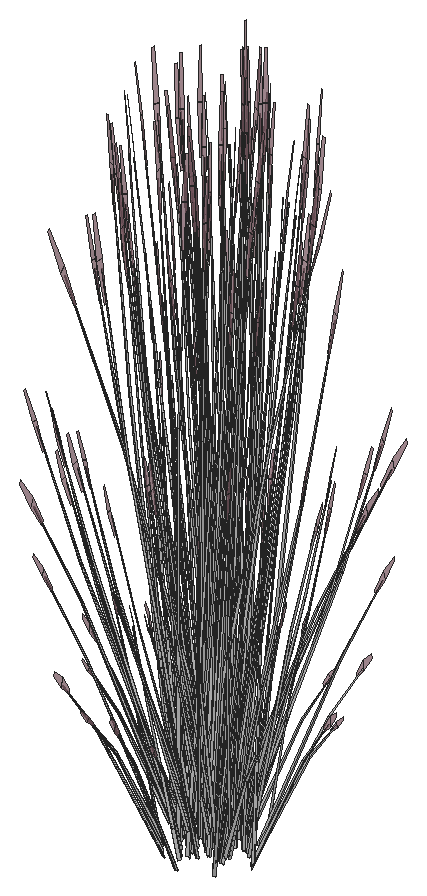
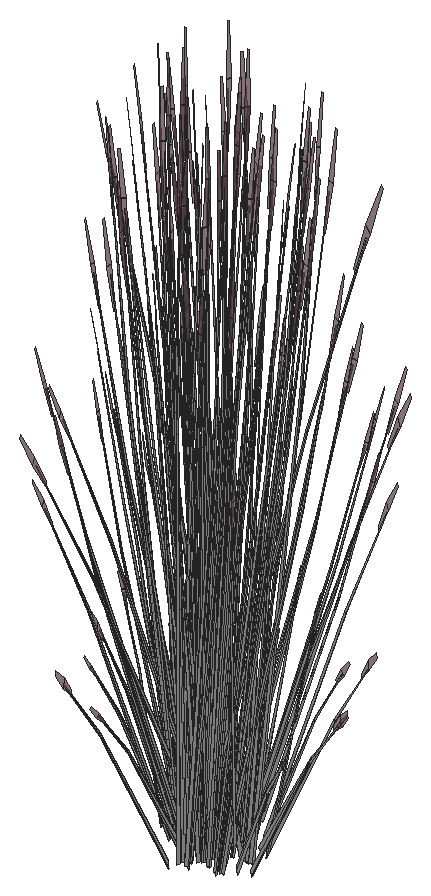
# SketchUp Ruby script. Lengths in inches.
U = 1.inch
M = Sketchup.active_model
def pt(a) = Geom::Point3d.new(a.map { |v| v * U })
def face(e, loops, mat)
  f = e.add_face(loops[0].map { |a| pt(a) })
  loops[1..].each { |l| e.add_face(l.map { |a| pt(a) }).erase! }
  f.material = f.back_material = mat if mat
  f
end
# faces: each face lists its corners as indices into pts; further lists are holes
def faces(e, pts, list, mat = nil) = list.each { |f| face(e, (f[0].is_a?(Array) ? f : [f]).map { |l| l.map { |i| pts[i] } }, mat) }
# xy, xz, yz: faces in a plane at the given z, y or x. An outline is a flat list of corners, or four numbers for a rectangle; further outlines are holes
def ring(l) = l.size == 4 ? [[l[0], l[1]], [l[2], l[1]], [l[2], l[3]], [l[0], l[3]]] : l.each_slice(2).to_a
def flat(e, list, mat, &to3) = list.each { |f| face(e, (f[0].is_a?(Array) ? f : [f]).map { |l| ring(l).map { |u, v| to3.(u, v) } }, mat) }
def xy(e, z, list, mat = nil) = flat(e, list, mat) { |x, y| [x, y, z] }
def xz(e, y, list, mat = nil) = flat(e, list, mat) { |x, z| [x, y, z] }
def yz(e, x, list, mat = nil) = flat(e, list, mat) { |y, z| [x, y, z] }
def lines(e, pts, list) = list.each { |a, b| e.add_line(pt(pts[a]), pt(pts[b])) }
# prism: a flat outline (further loops are holes) pulled along v
def prism(e, loops, v, mat = nil)
  f = face(e, loops, mat); d = Geom::Vector3d.new(v.map { |x| x * U })
  f.pushpull(f.normal.samedirection?(d) ? d.length : -d.length)
end
def box(e, o, s, mat = nil) = prism(e, [[o, [o[0] + s[0], o[1], o[2]], [o[0] + s[0], o[1] + s[1], o[2]], [o[0], o[1] + s[1], o[2]]]], [0, 0, s[2]], mat)
def at(x, y, z, deg = 0) = Geom::Transformation.translation(pt([x, y, z])) * Geom::Transformation.rotation(ORIGIN, Z_AXIS, deg.degrees)
def axes(o, x, y, z) = Geom::Transformation.new([*x, 0, *y, 0, *z, 0, *pt(o).to_a, 1])
def part(name) = M.definitions.add(name)
# library, detail: a bought-in or finely detailed component or shape, given as its bounding box
def library(name, o, s) = part(name).tap { |d| box(d.entities, o, s) }
def detail(e, o, s) = box(e.add_group.entities, o, s)
def put(e, d, t, mat = nil) = e.add_instance(d, t).tap { |i| i.material = mat if mat }
def group(e, t, mat = nil) = e.add_group.tap { |g| g.transformation = t; g.material = mat if mat }.entities
root = M.entities
M.materials.add("LightPink_Translucent").color = [144, 107, 117]
M.materials["LightPink_Translucent"].alpha = 0.75
M.materials.add("[_0053_Ivory_]").color = [200, 200, 200]
c1 = part("blade")
p = [[2.15,0.21,22],[0,0.17,0],[0.09,0.45,0],[2.18,0.31,22],[2.29,0.31,22],[0.38,0.45,0],
  [2.48,0.24,33],[2.49,0.24,33],[2.48,0.22,33]]
faces(c1.entities,p,[[0,1,2,3],[4,5,2,3],[6,3,4,7],[8,0,3,6]])
c2 = part("seeds")
p = [[0.3,-0.1,1.38],[-0.01,-0.03,1.59],[-0.01,-0.03,0.03],[0.14,-0.07,-0.07],[0.29,-0.03,3],[0.15,0.01,3.11]]
faces(c2.entities,p,[[0,1,2,3],[1,0,4,5]],"LightPink_Translucent")
c3 = part("blade with seeds")
put(c3.entities,c1,at(0,0,0))
put(c3.entities,c2,axes([2.4,0.25,30.99],[1.5799,-0.05474,1.17369],[-0.12525,1.92788,0.29478],[-0.07173,-0.02425,1.56792]))
put(root,c3,axes([642.49,106.9,130.53],[0.13883,0.2019,1.71376],[-0.64153,0.16998,0.13857],[-0.14499,-0.31697,0.73262]),"[_0053_Ivory_]")
put(root,c3,axes([644.98,106.61,129.24],[-0.17264,0.12729,1.43002],[-0.51703,-0.22279,-0.30754],[0.09584,-0.27707,0.61141]),"[_0053_Ivory_]")
put(root,c3,axes([644.2,107.05,131.63],[-0.28988,-0.51132,-0.71045],[0.59671,-0.28496,0.08574],[-0.06778,-0.24706,1.00501]),"[_0053_Ivory_]")
put(root,c3,axes([642.3125,106.37,129.24],[-0.03678,0.20572,1.43002],[-0.53767,0.17221,-0.30754],[-0.12568,-0.26589,0.61141]),"[_0053_Ivory_]")
put(root,c3,axes([643.7,105.92,128.15],[-0.10187,0.02266,1.76342],[-0.56336,-0.25503,-0.26939],[0.00945,-0.21273,0.30037]),"[_0053_Ivory_]")
put(root,c3,axes([645.4,107.55,131.63],[0.0158,-0.58168,-0.71045],[0.66548,0.03907,0.08574],[0.07023,-0.24643,1.00501]),"[_0053_Ivory_]")
put(root,c3,axes([644.25,106.62,131.18],[0.1831,-0.48359,-0.35414],[0.53419,0.14105,0.4572],[-0.04898,-0.1947,0.87481]),"[_0053_Ivory_]")
put(root,c3,axes([644.65,107.26,130.53],[-0.11309,0.21615,1.71376],[-0.47441,-0.44731,0.13857],[0.21402,-0.27879,0.73262]),"[_0053_Ivory_]")
put(root,c3,axes([643.98,106.95,131.33],[-0.59704,-0.15764,-0.51099],[0.20464,-0.54049,-0.3958],[-0.05475,-0.21761,0.97773]),"[_0053_Ivory_]")
put(root,c3,axes([644.35,105.59,129.42],[0.07791,0.3667,1.1486],[-0.43222,-0.2031,0.84392],[0.04651,-0.18776,0.25299]),"[_0053_Ivory_]")
put(root,c3,axes([645.27,107.36,131.33],[-0.43478,-0.42253,-0.51099],[0.45929,-0.37004,-0.3958],[0.06615,-0.21468,0.97773]),"[_0053_Ivory_]")
put(root,c3,axes([645.68,107.2,131.18],[0.41095,-0.33109,-0.35414],[0.38901,0.37805,0.4572],[0.05919,-0.19208,0.87481]),"[_0053_Ivory_]")
put(root,c3,axes([642.125,106.03,129.42],[0.31682,0.21887,1.1486],[-0.4614,0.13157,0.84392],[-0.09872,-0.16821,0.25299]),"[_0053_Ivory_]")
put(root,c3,axes([642.89,107.2,131.63],[-0.51789,-0.30395,-0.71045],[0.36805,-0.53263,0.08574],[-0.18764,-0.18149,1.00501]),"[_0053_Ivory_]")
put(root,c3,axes([642.71,106.79,131.18],[-0.0938,-0.50652,-0.35414],[0.53623,-0.13375,0.4572],[-0.14403,-0.14515,0.87481]),"[_0053_Ivory_]")
put(root,c3,axes([641.875,106.69,128.15],[-0.05883,0.08284,1.76342],[-0.59454,0.17861,-0.26939],[-0.14363,-0.16248,0.30037]),"[_0053_Ivory_]")
put(root,c3,axes([642.86,108.97,128.75],[-0.24943,-0.64486,-0.69835],[0.71849,-0.23224,-0.18329],[-0.02757,-0.21836,1.54149]),"[_0053_Ivory_]")
put(root,c3,axes([646.19,107,128.15],[-0.0909,-0.04954,1.76342],[-0.2335,-0.55347,-0.26939],[0.15752,-0.1502,0.30037]),"[_0053_Ivory_]")
put(root,c3,axes([642.65,107.21,131.33],[-0.59932,0.14948,-0.51099],[-0.10484,-0.56611,-0.3958],[-0.16097,-0.16223,0.97773]),"[_0053_Ivory_]")
put(root,c3,axes([646.1875,108.5625,131.63],[0.31725,-0.49618,-0.71045],[0.55593,0.35263,0.08574],[0.18942,-0.17977,1.00501]),"[_0053_Ivory_]")
put(root,c3,axes([642.76,107.12,129.03],[-0.37973,-0.63014,0],[0.6353,-0.35142,-0.51607],[0.14469,-0.08004,1.63711]),"[_0053_Ivory_]")
put(root,c3,axes([646.17,108.33,131.33],[-0.15602,-0.5742,-0.51099],[0.59087,-0.10045,-0.3958],[0.16933,-0.15423,0.97773]),"[_0053_Ivory_]")
put(root,c3,axes([643.59,106.36,128.78],[-0.4197,0.36076,-0.03893],[-0.38456,-0.39511,-0.17649],[-0.02707,-0.11196,0.58215]),"[_0053_Ivory_]")
put(root,c3,axes([644.13,110.63,129.98],[0.52485,0.25358,1.51261],[-0.51417,0.54629,0.59816],[-0.23031,-0.32378,1.26806]),"[_0053_Ivory_]")
put(root,c3,axes([641.39,108.88,128.67],[0,-0.62885,-0.49651],[0.67951,0,0],[0,-0.14322,1.57504]),"[_0053_Ivory_]")
put(root,c3,axes([643.27,107.02,128.67],[0.56842,-0.31443,-0.49651],[0.33976,0.56381,0],[0.12946,-0.07161,1.57504]),"[_0053_Ivory_]")
put(root,c3,axes([646.65,108.11,129.24],[-0.21697,-0.01863,1.43002],[-0.22228,-0.49966,-0.30754],[0.26655,-0.14135,0.61141]),"[_0053_Ivory_]")
put(root,c3,axes([643.95,108.31,128.71],[0.40909,-0.47266,-0.62353],[0.50819,0.4286,-0.16365],[0.16393,-0.11791,1.37633]),"[_0053_Ivory_]")
put(root,c3,axes([646.9,107.1875,129.42],[-0.2023,0.32011,1.1486],[-0.17388,-0.43009,0.84392],[0.16708,-0.10777,0.25299]),"[_0053_Ivory_]")
put(root,c3,axes([646.61,108.39,131.18],[0.52868,-0.08987,-0.35414],[0.1396,0.51376,0.4572],[0.1515,-0.13799,0.87481]),"[_0053_Ivory_]")
put(root,c3,axes([643.24,109.14,128.86],[0.29468,-0.56664,-0.44739],[0.61229,0.27271,0.21531],[0,-0.13062,1.43643]),"[_0053_Ivory_]")
put(root,c3,axes([641.47,107.68,131.18],[-0.34557,-0.39372,-0.35414],[0.39459,-0.37271,0.4572],[-0.20048,-0.05671,0.87481]),"[_0053_Ivory_]")
put(root,c3,axes([643.5,108.86,129.32],[-0.07077,-0.71755,-0.29095],[0.73712,-0.04339,-0.50002],[0.1298,-0.09558,1.59708]),"[_0053_Ivory_]")
put(root,c3,axes([641.68,108.89,128.68],[0.42396,-0.39235,-0.30978],[0.42396,0.39235,0.30978],[0,-0.12637,1.38974]),"[_0053_Ivory_]")
put(root,c3,axes([641.51,107.01,128.78],[-0.1752,0.51349,-0.03893],[-0.53924,-0.15795,-0.17649],[-0.08187,-0.08399,0.58215]),"[_0053_Ivory_]")
put(root,c3,axes([643.16,109.61,129.32],[-0.68399,-0.30005,-0.29095],[0.32934,-0.63331,-0.50002],[-0.0215,-0.15549,1.59708]),"[_0053_Ivory_]")
put(root,c3,axes([641.22,109.36,129.03],[-0.75945,0,0],[0,-0.70283,-0.51607],[0,-0.16007,1.63711]),"[_0053_Ivory_]")
put(root,c3,axes([643.41,107.27,128.68],[0.56663,0.1556,-0.30978],[-0.14267,0.54795,0.30978],[0.11423,-0.06319,1.38974]),"[_0053_Ivory_]")
put(root,c3,axes([641.8,109.17,128.98],[-0.56493,0.5287,0.30756],[-0.56528,-0.52313,-0.36492],[-0.01973,-0.15014,1.64885]),"[_0053_Ivory_]")
put(root,c3,axes([643.6,109.42,129.09],[0.68433,0.30479,0.24065],[-0.32934,0.63331,0.50002],[0,-0.14599,1.60543]),"[_0053_Ivory_]")
put(root,c3,axes([643.33,110.27,129.09],[0.16098,-0.74515,-0.23429],[0.76326,0.12989,0.51271],[-0.13337,-0.1029,1.5644]),"[_0053_Ivory_]")
put(root,c3,axes([640.64,108.63,129.42],[0.38775,-0.045,1.1486],[-0.24596,0.39648,0.84392],[-0.19161,-0.05948,0.25299]),"[_0053_Ivory_]")
put(root,c3,axes([643.38,108.99,129.37],[-0.65953,0.03882,0.44739],[-0.05964,-0.64439,-0.21531],[0.11807,-0.06531,1.43643]),"[_0053_Ivory_]")
put(root,c3,axes([641.68,109.46,129.13],[0,0.62885,0.49651],[-0.67951,0,0],[0,-0.14322,1.57504]),"[_0053_Ivory_]")
put(root,c3,axes([646.45,109.6,131.33],[0.16454,-0.57202,-0.51099],[0.56413,0.19607,-0.3958],[0.22713,-0.05245,0.97773]),"[_0053_Ivory_]")
put(root,c3,axes([645.55,107.28,129.03],[0.37973,-0.63014,0],[0.6353,0.35142,-0.51607],[0.14469,0.08004,1.63711]),"[_0053_Ivory_]")
put(root,c3,axes([643.28,109.97,128.86],[-0.36485,-0.52782,-0.44739],[0.55265,-0.37168,0.21531],[-0.11807,-0.06531,1.43643]),"[_0053_Ivory_]")
put(root,c3,axes([643.36,109.23,129.01],[0.26406,0.70318,0.45755],[-0.7545,0.24452,0.17955],[0.00922,-0.12921,1.58856]),"[_0053_Ivory_]")
put(root,c3,axes([647.05,109.77,128.64],[-0.39118,0.07547,1.41583],[-0.06226,-0.6007,0.08104],[0.27398,-0.09092,0.80566]),"[_0053_Ivory_]")
put(root,c3,axes([647.76,109.23,128.91],[-0.37654,-0.40212,-0.06488],[0.4124,-0.36845,-0.29416],[0.11685,-0.02594,0.97024]),"[_0053_Ivory_]")
put(root,c3,axes([643.22,109.78,129.37],[-0.29468,0.56664,0.44739],[-0.61229,-0.27271,-0.21531],[0,-0.13062,1.43643]),"[_0053_Ivory_]")
put(root,c3,axes([644.31,109.29,128.86],[0,-0.72763,0],[0.75945,0,0],[0,0,1.79456]),"[_0053_Ivory_]")
put(root,c3,axes([645.23,107.6,129.13],[-0.56842,-0.31443,0.49651],[0.33976,-0.56381,0],[0.12946,0.07161,1.57504]),"[_0053_Ivory_]")
put(root,c3,axes([646.34,109.8125,131.63],[0.53369,-0.27773,-0.71045],[0.29743,0.5717,0.08574],[0.25786,-0.06494,1.00501]),"[_0053_Ivory_]")
put(root,c3,axes([642.95,110.17,128.71],[-0.63179,-0.1031,-0.62353],[0.13332,-0.63596,-0.16365],[-0.18854,-0.07706,1.37633]),"[_0053_Ivory_]")
put(root,c3,axes([643.95,108.83,129.01],[-0.50358,0.57069,0.45755],[-0.59827,-0.50377,0.17955],[0.1214,-0.05695,1.58856]),"[_0053_Ivory_]")
put(root,c3,axes([644.5,109.85,128.95],[-0.56493,-0.54126,-0.06131],[0.56528,-0.54159,0],[-0.01973,-0.0189,1.75571]),"[_0053_Ivory_]")
put(root,c3,axes([643.07,107.89,129.13],[-0.17545,0.62497,0.17642],[-0.64204,-0.17686,0.35086],[0.11091,-0.00304,1.60407]),"[_0053_Ivory_]")
put(root,c3,axes([642.81,108.39,128.25],[-0.59782,0.25177,1.28929],[-0.19028,-0.72239,0.50096],[0.36709,0.01202,1.46642]),"[_0053_Ivory_]")
put(root,c3,axes([644.41,108.58,129.27],[0.11717,-0.56122,0.1448],[0.57245,0.09742,-0.41347],[0.10418,0.05763,1.26744]),"[_0053_Ivory_]")
put(root,c3,axes([643.42,109.92,129.01],[0.76764,0.13249,0.45755],[-0.15622,0.74829,0.17955],[-0.11218,-0.07226,1.58856]),"[_0053_Ivory_]")
put(root,c3,axes([647.48,109.375,128.15],[-0.03174,-0.09547,1.76342],[0.22015,-0.55846,-0.26939],[0.22208,-0.00803,0.30037]),"[_0053_Ivory_]")
put(root,c3,axes([640.92,109.28,128.15],[0.0154,0.09911,1.76342],[-0.31051,0.51756,-0.26939],[-0.22056,-0.02609,0.30037]),"[_0053_Ivory_]")
put(root,c3,axes([644.17,108.73,129.37],[-0.36485,-0.52782,0.44739],[0.55265,-0.37168,-0.21531],[0.11807,0.06531,1.43643]),"[_0053_Ivory_]")
put(root,c3,axes([642.28,111.14,128.68],[-0.14267,-0.54795,-0.30978],[0.56663,-0.1556,0.30978],[-0.11423,-0.06319,1.38974]),"[_0053_Ivory_]")
put(root,c3,axes([643.01,111.11,129.13],[0.65264,-0.16691,0.17642],[0.16115,0.62115,0.35086],[-0.05821,-0.0905,1.60407]),"[_0053_Ivory_]")
put(root,c3,axes([644.35,108.76,129.32],[0.61322,-0.4175,-0.29095],[0.40778,0.58992,-0.50002],[0.1513,0.05991,1.59708]),"[_0053_Ivory_]")
put(root,c3,axes([646.79,109.87,131.18],[0.50475,0.17543,-0.35414],[-0.14722,0.5118,0.4572],[0.20322,-0.04693,0.87481]),"[_0053_Ivory_]")
put(root,c3,axes([642.125,111.38,128.67],[-0.56842,-0.31443,-0.49651],[0.33976,-0.56381,0],[-0.12946,-0.07161,1.57504]),"[_0053_Ivory_]")
put(root,c3,axes([645.9,107.66,128.67],[0.56842,0.31443,-0.49651],[-0.33976,0.56381,0],[0.12946,0.07161,1.57504]),"[_0053_Ivory_]")
put(root,c3,axes([644.82,109.45,128.86],[0.67951,0,0],[0,0.65103,0],[0,0,1.78407]),"[_0053_Ivory_]")
put(root,c3,axes([643.67,110.27,129.32],[-0.61322,0.4175,-0.29095],[-0.40778,-0.58992,-0.50002],[-0.1513,-0.05991,1.59708]),"[_0053_Ivory_]")
put(root,c3,axes([645.01,107.92,129.13],[-0.65264,0.16691,0.17642],[-0.16115,-0.62115,0.35086],[0.05821,0.0905,1.60407]),"[_0053_Ivory_]")
put(root,c3,axes([645.42,109.23,130.53],[-0.25192,0.01424,1.71376],[0.16712,-0.61729,0.13857],[0.35901,0.03818,0.73262]),"[_0053_Ivory_]")
put(root,c3,axes([645.74,107.89,128.68],[0.14267,0.54795,-0.30978],[-0.56663,0.1556,0.30978],[0.11423,0.06319,1.38974]),"[_0053_Ivory_]")
put(root,c3,axes([644.6,109.12,129.03],[-0.76764,-0.13249,0.49198],[0.15622,-0.74829,0.19306],[0.11218,0.07226,1.70813]),"[_0053_Ivory_]")
put(root,c3,axes([643.99,110.96,128.86],[-0.19817,-0.54216,0],[0.56587,-0.18986,0],[0,0,1.54371]),"[_0053_Ivory_]")
put(root,c3,axes([643.61,110.45,129.27],[-0.11717,0.56122,0.1448],[-0.57245,-0.09742,-0.41347],[-0.10418,-0.05763,1.26744]),"[_0053_Ivory_]")
put(root,c3,axes([644.73,110.89,128.84],[0.63764,-0.21337,-0.19198],[0.22406,0.61462,0.00008],[0.07038,-0.02358,1.73897]),"[_0053_Ivory_]")
put(root,c3,axes([644.95,111.15,129.13],[0.17545,-0.62497,0.17642],[0.64204,0.17686,0.35086],[-0.11091,0.00304,1.60407]),"[_0053_Ivory_]")
put(root,c3,axes([644.81,109.73,128.87],[0.42396,0.40619,0],[-0.42396,0.40619,0],[0,0,1.69266]),"[_0053_Ivory_]")
put(root,c3,axes([645.95,109.55,129.13],[-0.47719,-0.45806,0.17642],[0.48088,-0.44429,0.35086],[-0.0527,0.09355,1.60407]),"[_0053_Ivory_]")
put(root,c3,axes([645.07,108.86,128.71],[0.63179,0.1031,-0.62353],[-0.13332,0.63596,-0.16365],[0.18854,0.07706,1.37633]),"[_0053_Ivory_]")
put(root,c3,axes([647.86,109.97,129.42],[-0.37526,0.10382,1.1486],[0.17664,-0.42906,0.84392],[0.19907,0.02936,0.25299]),"[_0053_Ivory_]")
put(root,c3,axes([643.85,111.21,128.85],[-0.61229,-0.28233,0],[0.29468,-0.58663,0],[0,0,1.62707]),"[_0053_Ivory_]")
put(root,c3,axes([644.36,110.46,129.12],[-0.59306,-0.50614,-0.25192],[0.49904,-0.56836,0.5513],[-0.1597,0.05921,1.68216]),"[_0053_Ivory_]")
put(root,c3,axes([642.8,111.43,129.13],[0.56842,0.31443,0.49651],[-0.33976,0.56381,0],[-0.12946,-0.07161,1.57504]),"[_0053_Ivory_]")
put(root,c3,axes([644.8,109.25,129.37],[0.29468,-0.56664,0.44739],[0.61229,0.27271,-0.21531],[0,0.13062,1.43643]),"[_0053_Ivory_]")
put(root,c3,axes([644.6875,109.58,128.95],[0,0.72727,-0.05637],[-0.75945,0,0],[0,0.02286,1.79368]),"[_0053_Ivory_]")
put(root,c3,axes([644.74,109.0625,128.86],[0.36485,0.52782,-0.44739],[-0.55265,0.37168,0.21531],[0.11807,0.06531,1.43643]),"[_0053_Ivory_]")
put(root,c3,axes([647.21,111.29,130.58],[-0.11624,-0.52862,-0.03492],[0.54943,-0.12153,-0.15832],[0.11473,0.03351,0.52218]),"[_0053_Ivory_]")
put(root,c3,axes([642.47,111.76,129.03],[-0.37973,0.63014,0],[-0.6353,-0.35142,-0.51607],[-0.14469,-0.08004,1.63711]),"[_0053_Ivory_]")
put(root,c3,axes([646.35,109.57,129.13],[0,-0.62885,0.49651],[0.67951,0,0],[0,0.14322,1.57504]),"[_0053_Ivory_]")
put(root,c3,axes([644.65,110.04,129.37],[0.65953,-0.03882,0.44739],[0.05964,0.64439,-0.21531],[-0.11807,0.06531,1.43643]),"[_0053_Ivory_]")
put(root,c3,axes([645.06,109.38,129.27],[0.56587,-0.18339,0.1448],[0.19817,0.52368,-0.41347],[0,0.11525,1.26744]),"[_0053_Ivory_]")
put(root,c3,axes([644.06,110.35,128.86],[-0.65953,0.03882,-0.44739],[-0.05964,-0.64439,0.21531],[-0.11807,0.06531,1.43643]),"[_0053_Ivory_]")
put(root,c3,axes([647.16,110.66,129.24],[-0.14627,-0.15466,1.43002],[0.19032,-0.51164,-0.30754],[0.29594,0.06931,0.61141]),"[_0053_Ivory_]")
put(root,c3,axes([644.55,111.22,128.86],[0.61229,0.28233,0],[-0.29468,0.58663,0],[0,0,1.74954]),"[_0053_Ivory_]")
put(root,c3,axes([644.79,111.85,128.85],[-0.37499,-0.63235,-0.05142],[0.6353,-0.35142,0.51607],[-0.15655,0.0602,1.6363]),"[_0053_Ivory_]")
put(root,c3,axes([644.66,110.32,129.27],[0.44871,0.37783,0.1448],[-0.37428,0.42627,-0.41347],[-0.10418,0.05763,1.26744]),"[_0053_Ivory_]")
put(root,c3,axes([645.82,110.97,131.63],[0.60713,0.01514,-0.71045],[-0.04078,0.63759,0.08574],[0.25721,0.06729,1.00501]),"[_0053_Ivory_]")
put(root,c3,axes([645.13,111.48,129.13],[0.56842,-0.31443,0.49651],[0.33976,0.56381,0],[-0.12946,0.07161,1.57504]),"[_0053_Ivory_]")
put(root,c3,axes([644.32,110.98,128.94],[0.26406,0.72244,-0.06012],[-0.7545,0.25315,0],[0.00922,0.02523,1.72173]),"[_0053_Ivory_]")
put(root,c3,axes([644.62,111.77,128.68],[-0.56663,-0.1556,-0.30978],[0.14267,-0.54795,0.30978],[-0.11423,0.06319,1.38974]),"[_0053_Ivory_]")
put(root,c3,axes([646.81,109.68,129.03],[0.75945,0,0],[0,0.70283,-0.51607],[0,0.16007,1.63711]),"[_0053_Ivory_]")
put(root,c3,axes([646.51,110.04,128.85],[-0.75908,-0.00503,-0.04976],[0,-0.70283,0.49943],[-0.02386,0.16,1.58352]),"[_0053_Ivory_]")
put(root,c3,axes([644.86,109.42,129.32],[0.68399,0.30005,-0.29095],[-0.32934,0.63331,-0.50002],[0.0215,0.15549,1.59708]),"[_0053_Ivory_]")
put(root,c3,axes([640.09,111.76,129.42],[0.25312,-0.28501,1.1486],[0.09988,0.45119,0.84392],[-0.18292,0.08079,0.25299]),"[_0053_Ivory_]")
put(root,c3,axes([646.18,111.23,131.18],[0.34557,0.39372,-0.35414],[-0.39459,0.37271,0.4572],[0.20048,0.05671,0.87481]),"[_0053_Ivory_]")
put(root,c3,axes([646.35,110.14,128.68],[-0.42396,0.39235,-0.30978],[-0.42396,-0.39235,0.30978],[0,0.12637,1.38974]),"[_0053_Ivory_]")
put(root,c3,axes([644.52,110.18,129.32],[0.07077,0.71755,-0.29095],[-0.73712,0.04339,-0.50002],[-0.1298,0.09558,1.59708]),"[_0053_Ivory_]")
put(root,c3,axes([644.79,109.9,128.86],[-0.29468,0.56664,-0.44739],[-0.61229,-0.27271,0.21531],[0,0.13062,1.43643]),"[_0053_Ivory_]")
put(root,c3,axes([641.04,110.53,131.18],[-0.52868,0.08987,-0.35414],[-0.1396,-0.51376,0.4572],[-0.1515,0.13799,0.87481]),"[_0053_Ivory_]")
put(root,c3,axes([644.08,110.72,128.71],[-0.40909,0.47266,-0.62353],[-0.50819,-0.4286,-0.16365],[-0.16393,0.11791,1.37633]),"[_0053_Ivory_]")
put(root,c3,axes([644.81,111.52,128.98],[0.76036,0.2044,0.30756],[-0.19023,0.7306,-0.36492],[-0.12585,0.09144,1.64885]),"[_0053_Ivory_]")
put(root,c3,axes([644.75,112.01,128.67],[-0.56842,0.31443,-0.49651],[-0.33976,-0.56381,0],[-0.12946,0.07161,1.57504]),"[_0053_Ivory_]")
put(root,c3,axes([646.64,110.15,128.67],[0,0.62885,-0.49651],[-0.67951,0,0],[0,0.14322,1.57504]),"[_0053_Ivory_]")
put(root,c3,axes([644.94,110.22,130.53],[-0.2256,-0.10835,1.71376],[0.46687,-0.45453,0.13857],[0.29098,0.20505,0.73262]),"[_0053_Ivory_]")
put(root,c3,axes([645.78,111.46,129.42],[-0.34197,-0.18082,1.1486],[0.44156,-0.18372,0.84392],[0.1191,0.15563,0.25299]),"[_0053_Ivory_]")
put(root,c3,axes([641.96,110.02,130.53],[0.1517,-0.19322,1.71376],[0.38303,0.52154,0.13857],[-0.26271,0.23751,0.73262]),"[_0053_Ivory_]")
put(root,c3,axes([641.48,110.59,131.33],[0.15602,0.5742,-0.51099],[-0.59087,0.10045,-0.3958],[-0.16933,0.15423,0.97773]),"[_0053_Ivory_]")
put(root,c3,axes([645.27,111.92,129.03],[0.37973,0.63014,0],[-0.6353,0.35142,-0.51607],[-0.14469,0.08004,1.63711]),"[_0053_Ivory_]")
put(root,c3,axes([645.87,112.13,128.15],[0.04425,-0.09079,1.76342],[0.55709,-0.26738,-0.26939],[0.16889,0.13839,0.30037]),"[_0053_Ivory_]")
put(root,c3,axes([644.94,109.42,129.5],[-0.01659,-0.59209,1.41272],[0.75089,0.15348,0.59816],[-0.1776,0.32398,1.3335]),"[_0053_Ivory_]")
put(root,c3,axes([645.14,110.07,128.75],[0.2227,0.57576,-0.69212],[-0.64151,0.20736,-0.18165],[0.02462,0.19497,1.52773]),"[_0053_Ivory_]")
